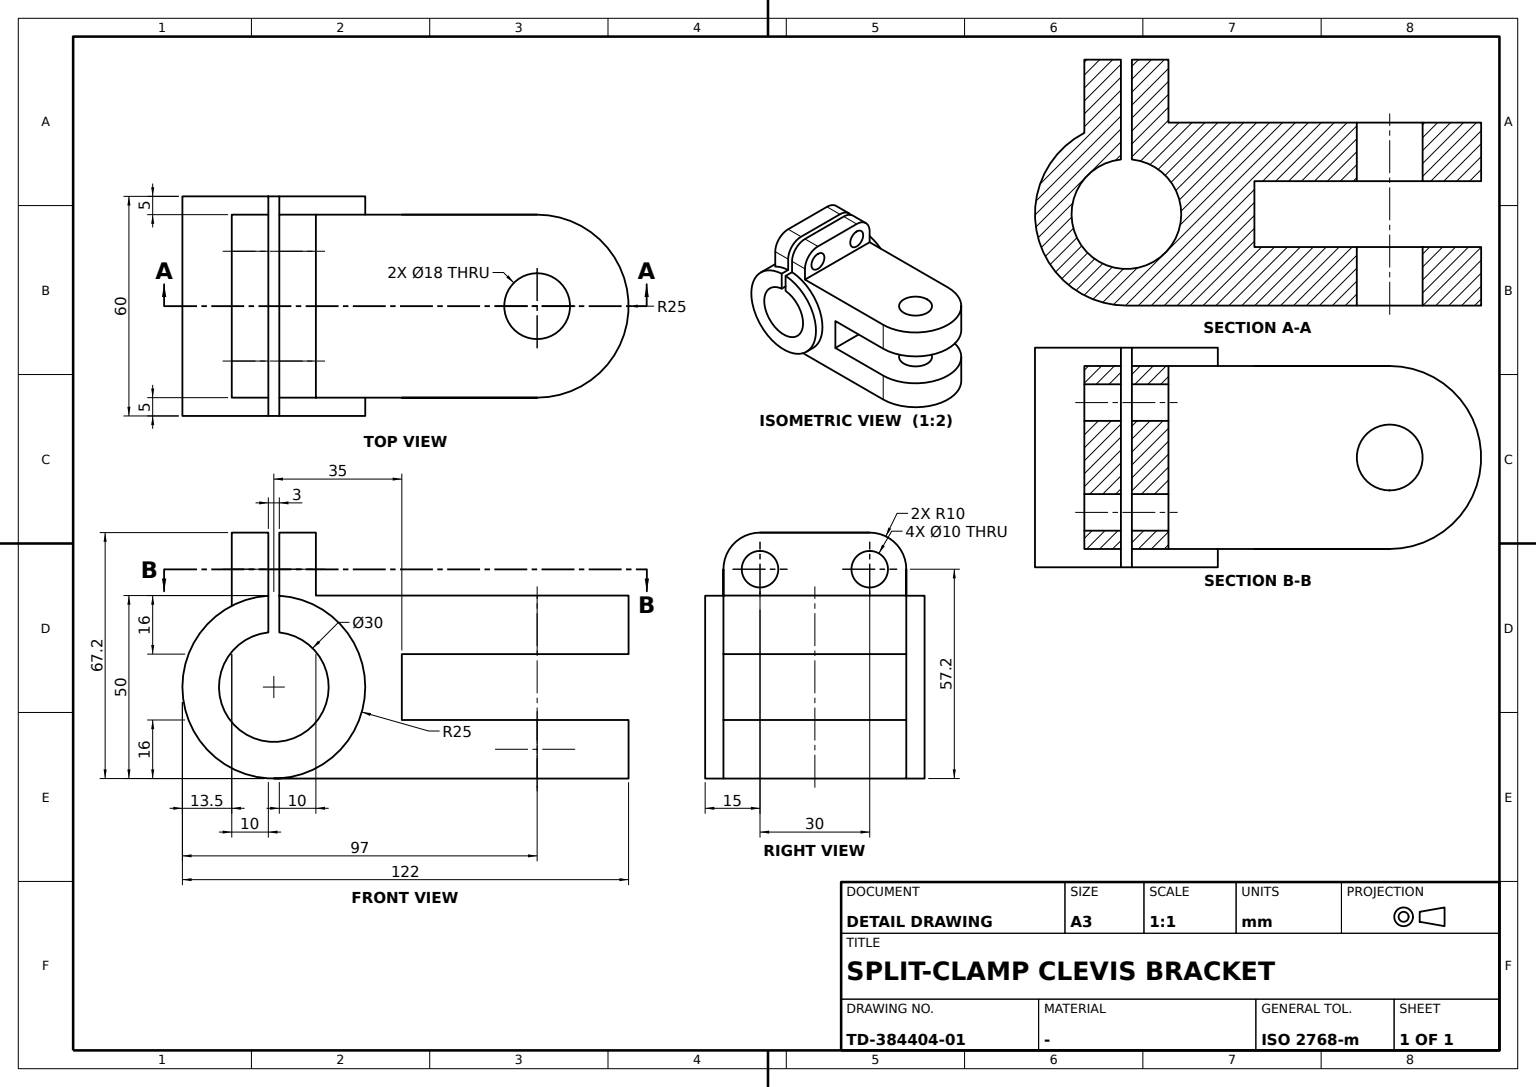
ISO-10303-21;
HEADER;
FILE_DESCRIPTION((''),'2;1');
FILE_NAME('','',(''),(''),'','','');
FILE_SCHEMA(('AUTOMOTIVE_DESIGN'));
ENDSEC;
DATA;
#1=APPLICATION_CONTEXT('');
#2=PRODUCT_CONTEXT('',#1,'mechanical');
#3=PRODUCT('','','',(#2));
#4=PRODUCT_DEFINITION_FORMATION('','',#3);
#5=PRODUCT_DEFINITION_CONTEXT('',#1,'design');
#6=PRODUCT_DEFINITION('','',#4,#5);
#7=PRODUCT_DEFINITION_SHAPE('','',#6);
#8=(LENGTH_UNIT()NAMED_UNIT(*)SI_UNIT(.MILLI.,.METRE.));
#9=(NAMED_UNIT(*)PLANE_ANGLE_UNIT()SI_UNIT($,.RADIAN.));
#10=(NAMED_UNIT(*)SI_UNIT($,.STERADIAN.)SOLID_ANGLE_UNIT());
#11=UNCERTAINTY_MEASURE_WITH_UNIT(LENGTH_MEASURE(0.005),#8,'distance_accuracy_value','');
#12=(GEOMETRIC_REPRESENTATION_CONTEXT(3)GLOBAL_UNCERTAINTY_ASSIGNED_CONTEXT((#11))GLOBAL_UNIT_ASSIGNED_CONTEXT((#8,#9,#10))REPRESENTATION_CONTEXT('',''));
#13=CARTESIAN_POINT('',(9.,72.,-25.));
#14=VERTEX_POINT('',#13);
#15=CARTESIAN_POINT('',(0.,72.,-25.));
#16=DIRECTION('',(0.,0.,1.));
#17=DIRECTION('',(1.,0.,0.));
#18=AXIS2_PLACEMENT_3D('',#15,#16,#17);
#19=CIRCLE('',#18,9.);
#20=EDGE_CURVE('',#14,#14,#19,.T.);
#21=ORIENTED_EDGE('',*,*,#20,.T.);
#22=EDGE_LOOP('',(#21));
#23=FACE_BOUND('',#22,.T.);
#24=CARTESIAN_POINT('',(-25.,0.,-25.));
#25=VERTEX_POINT('',#24);
#26=CARTESIAN_POINT('',(25.,0.,-25.));
#27=VERTEX_POINT('',#26);
#28=CARTESIAN_POINT('',(0.,0.,-25.));
#29=VECTOR('',#17,1000.);
#30=LINE('',#28,#29);
#31=EDGE_CURVE('',#25,#27,#30,.T.);
#32=ORIENTED_EDGE('',*,*,#31,.F.);
#33=CARTESIAN_POINT('',(-25.,72.,-25.));
#34=VERTEX_POINT('',#33);
#35=DIRECTION('',(0.,-1.,0.));
#36=VECTOR('',#35,1000.);
#37=LINE('',#24,#36);
#38=EDGE_CURVE('',#34,#25,#37,.T.);
#39=ORIENTED_EDGE('',*,*,#38,.F.);
#40=CARTESIAN_POINT('',(25.,72.,-25.));
#41=VERTEX_POINT('',#40);
#42=CIRCLE('',#18,25.);
#43=EDGE_CURVE('',#41,#34,#42,.T.);
#44=ORIENTED_EDGE('',*,*,#43,.F.);
#45=LINE('',#26,#36);
#46=EDGE_CURVE('',#41,#27,#45,.T.);
#47=ORIENTED_EDGE('',*,*,#46,.T.);
#48=EDGE_LOOP('',(#32,#39,#44,#47));
#49=FACE_BOUND('',#48,.T.);
#50=CARTESIAN_POINT('',(0.,97.,-25.));
#51=AXIS2_PLACEMENT_3D('',#50,#16,#35);
#52=PLANE('',#51);
#53=ADVANCED_FACE('',(#23,#49),#52,.F.);
#54=CARTESIAN_POINT('',(25.,-1.5,24.954959));
#55=VERTEX_POINT('',#54);
#56=CARTESIAN_POINT('',(25.,-11.5,22.197973));
#57=VERTEX_POINT('',#56);
#58=CARTESIAN_POINT('',(25.,0.,0.));
#59=DIRECTION('',(0.,0.,-1.));
#60=AXIS2_PLACEMENT_3D('',#58,#17,#59);
#61=CIRCLE('',#60,25.);
#62=EDGE_CURVE('',#55,#57,#61,.T.);
#63=ORIENTED_EDGE('',*,*,#62,.F.);
#64=CARTESIAN_POINT('',(25.,-1.5,32.197973));
#65=VERTEX_POINT('',#64);
#66=CARTESIAN_POINT('',(25.,-1.5,0.));
#67=VECTOR('',#16,1000.);
#68=LINE('',#66,#67);
#69=EDGE_CURVE('',#55,#65,#68,.T.);
#70=ORIENTED_EDGE('',*,*,#69,.T.);
#71=CARTESIAN_POINT('',(25.,-11.5,32.197973));
#72=VERTEX_POINT('',#71);
#73=CARTESIAN_POINT('',(25.,-6.5,32.197973));
#74=DIRECTION('',(0.,1.,0.));
#75=VECTOR('',#74,1000.);
#76=LINE('',#73,#75);
#77=EDGE_CURVE('',#72,#65,#76,.T.);
#78=ORIENTED_EDGE('',*,*,#77,.F.);
#79=CARTESIAN_POINT('',(25.,-11.5,0.));
#80=VECTOR('',#59,1000.);
#81=LINE('',#79,#80);
#82=EDGE_CURVE('',#72,#57,#81,.T.);
#83=ORIENTED_EDGE('',*,*,#82,.T.);
#84=EDGE_LOOP('',(#63,#70,#78,#83));
#85=FACE_BOUND('',#84,.T.);
#86=AXIS2_PLACEMENT_3D('',#58,#17,#74);
#87=PLANE('',#86);
#88=ADVANCED_FACE('',(#85),#87,.T.);
#89=ORIENTED_EDGE('',*,*,#46,.F.);
#90=CARTESIAN_POINT('',(25.,72.,-9.));
#91=VERTEX_POINT('',#90);
#92=CARTESIAN_POINT('',(25.,72.,8.598986));
#93=LINE('',#92,#80);
#94=EDGE_CURVE('',#91,#41,#93,.T.);
#95=ORIENTED_EDGE('',*,*,#94,.F.);
#96=CARTESIAN_POINT('',(25.,35.,-9.));
#97=VERTEX_POINT('',#96);
#98=CARTESIAN_POINT('',(25.,0.,-9.));
#99=LINE('',#98,#75);
#100=EDGE_CURVE('',#97,#91,#99,.T.);
#101=ORIENTED_EDGE('',*,*,#100,.F.);
#102=CARTESIAN_POINT('',(25.,35.,9.));
#103=VERTEX_POINT('',#102);
#104=CARTESIAN_POINT('',(25.,35.,0.));
#105=LINE('',#104,#80);
#106=EDGE_CURVE('',#103,#97,#105,.T.);
#107=ORIENTED_EDGE('',*,*,#106,.F.);
#108=CARTESIAN_POINT('',(25.,72.,9.));
#109=VERTEX_POINT('',#108);
#110=CARTESIAN_POINT('',(25.,0.,9.));
#111=LINE('',#110,#36);
#112=EDGE_CURVE('',#109,#103,#111,.T.);
#113=ORIENTED_EDGE('',*,*,#112,.F.);
#114=CARTESIAN_POINT('',(25.,72.,25.));
#115=VERTEX_POINT('',#114);
#116=EDGE_CURVE('',#115,#109,#93,.T.);
#117=ORIENTED_EDGE('',*,*,#116,.F.);
#118=CARTESIAN_POINT('',(25.,11.5,25.));
#119=VERTEX_POINT('',#118);
#120=CARTESIAN_POINT('',(25.,0.,25.));
#121=LINE('',#120,#75);
#122=EDGE_CURVE('',#119,#115,#121,.T.);
#123=ORIENTED_EDGE('',*,*,#122,.F.);
#124=CARTESIAN_POINT('',(25.,11.5,32.197973));
#125=VERTEX_POINT('',#124);
#126=CARTESIAN_POINT('',(25.,11.5,0.));
#127=LINE('',#126,#80);
#128=EDGE_CURVE('',#125,#119,#127,.T.);
#129=ORIENTED_EDGE('',*,*,#128,.F.);
#130=CARTESIAN_POINT('',(25.,1.5,32.197969));
#131=VERTEX_POINT('',#130);
#132=EDGE_CURVE('',#125,#131,#76,.F.);
#133=ORIENTED_EDGE('',*,*,#132,.T.);
#134=CARTESIAN_POINT('',(25.,1.5,24.954959));
#135=VERTEX_POINT('',#134);
#136=CARTESIAN_POINT('',(25.,1.5,0.));
#137=LINE('',#136,#67);
#138=EDGE_CURVE('',#135,#131,#137,.T.);
#139=ORIENTED_EDGE('',*,*,#138,.F.);
#140=EDGE_CURVE('',#27,#135,#61,.T.);
#141=ORIENTED_EDGE('',*,*,#140,.F.);
#142=EDGE_LOOP('',(#89,#95,#101,#107,#113,#117,#123,#129,#133,#139,#141));
#143=FACE_BOUND('',#142,.T.);
#144=ADVANCED_FACE('',(#143),#87,.T.);
#145=ORIENTED_EDGE('',*,*,#94,.T.);
#146=ORIENTED_EDGE('',*,*,#43,.T.);
#147=CARTESIAN_POINT('',(-25.,72.,-9.));
#148=VERTEX_POINT('',#147);
#149=CARTESIAN_POINT('',(-25.,72.,8.598986));
#150=LINE('',#149,#80);
#151=EDGE_CURVE('',#148,#34,#150,.T.);
#152=ORIENTED_EDGE('',*,*,#151,.F.);
#153=CARTESIAN_POINT('',(0.,72.,-9.));
#154=DIRECTION('',(-1.,0.,0.));
#155=AXIS2_PLACEMENT_3D('',#153,#59,#154);
#156=CIRCLE('',#155,25.);
#157=EDGE_CURVE('',#148,#91,#156,.T.);
#158=ORIENTED_EDGE('',*,*,#157,.T.);
#159=EDGE_LOOP('',(#145,#146,#152,#158));
#160=FACE_BOUND('',#159,.T.);
#161=CARTESIAN_POINT('',(0.,72.,8.598986));
#162=AXIS2_PLACEMENT_3D('',#161,#59,#74);
#163=CYLINDRICAL_SURFACE('',#162,25.);
#164=ADVANCED_FACE('',(#160),#163,.T.);
#165=CARTESIAN_POINT('',(-25.,35.,9.));
#166=VERTEX_POINT('',#165);
#167=CARTESIAN_POINT('',(-25.,35.,-9.));
#168=VERTEX_POINT('',#167);
#169=CARTESIAN_POINT('',(-25.,35.,0.));
#170=LINE('',#169,#80);
#171=EDGE_CURVE('',#166,#168,#170,.T.);
#172=ORIENTED_EDGE('',*,*,#171,.F.);
#173=CARTESIAN_POINT('',(0.,35.,9.));
#174=LINE('',#173,#29);
#175=EDGE_CURVE('',#166,#103,#174,.T.);
#176=ORIENTED_EDGE('',*,*,#175,.T.);
#177=ORIENTED_EDGE('',*,*,#106,.T.);
#178=CARTESIAN_POINT('',(0.,35.,-9.));
#179=LINE('',#178,#29);
#180=EDGE_CURVE('',#168,#97,#179,.T.);
#181=ORIENTED_EDGE('',*,*,#180,.F.);
#182=EDGE_LOOP('',(#172,#176,#177,#181));
#183=FACE_BOUND('',#182,.T.);
#184=AXIS2_PLACEMENT_3D('',#173,#35,#59);
#185=PLANE('',#184);
#186=ADVANCED_FACE('',(#183),#185,.F.);
#187=CARTESIAN_POINT('',(-15.,-11.5,42.197973));
#188=VERTEX_POINT('',#187);
#189=CARTESIAN_POINT('',(15.,-11.5,42.197973));
#190=VERTEX_POINT('',#189);
#191=CARTESIAN_POINT('',(0.,-11.5,42.197973));
#192=LINE('',#191,#29);
#193=EDGE_CURVE('',#188,#190,#192,.T.);
#194=ORIENTED_EDGE('',*,*,#193,.T.);
#195=CARTESIAN_POINT('',(15.,-1.5,42.197973));
#196=VERTEX_POINT('',#195);
#197=CARTESIAN_POINT('',(15.,-6.5,42.197973));
#198=LINE('',#197,#75);
#199=EDGE_CURVE('',#190,#196,#198,.T.);
#200=ORIENTED_EDGE('',*,*,#199,.T.);
#201=CARTESIAN_POINT('',(-15.,-1.5,42.197973));
#202=VERTEX_POINT('',#201);
#203=CARTESIAN_POINT('',(0.,-1.5,42.197973));
#204=LINE('',#203,#29);
#205=EDGE_CURVE('',#202,#196,#204,.T.);
#206=ORIENTED_EDGE('',*,*,#205,.F.);
#207=CARTESIAN_POINT('',(-15.,-6.5,42.197973));
#208=LINE('',#207,#36);
#209=EDGE_CURVE('',#202,#188,#208,.T.);
#210=ORIENTED_EDGE('',*,*,#209,.T.);
#211=EDGE_LOOP('',(#194,#200,#206,#210));
#212=FACE_BOUND('',#211,.T.);
#213=AXIS2_PLACEMENT_3D('',#203,#16,#35);
#214=PLANE('',#213);
#215=ADVANCED_FACE('',(#212),#214,.T.);
#216=CARTESIAN_POINT('',(-15.,11.5,27.197973));
#217=VERTEX_POINT('',#216);
#218=CARTESIAN_POINT('',(-15.,11.5,32.197973));
#219=AXIS2_PLACEMENT_3D('',#218,#35,#59);
#220=CIRCLE('',#219,5.);
#221=EDGE_CURVE('',#217,#217,#220,.F.);
#222=ORIENTED_EDGE('',*,*,#221,.F.);
#223=EDGE_LOOP('',(#222));
#224=FACE_BOUND('',#223,.T.);
#225=CARTESIAN_POINT('',(-25.,11.5,32.197969));
#226=VERTEX_POINT('',#225);
#227=CARTESIAN_POINT('',(-25.,11.5,25.));
#228=VERTEX_POINT('',#227);
#229=CARTESIAN_POINT('',(-25.,11.5,0.));
#230=LINE('',#229,#80);
#231=EDGE_CURVE('',#226,#228,#230,.T.);
#232=ORIENTED_EDGE('',*,*,#231,.F.);
#233=CARTESIAN_POINT('',(-15.,11.5,42.197973));
#234=VERTEX_POINT('',#233);
#235=CIRCLE('',#219,10.);
#236=EDGE_CURVE('',#234,#226,#235,.T.);
#237=ORIENTED_EDGE('',*,*,#236,.F.);
#238=CARTESIAN_POINT('',(14.999996,11.5,42.197973));
#239=VERTEX_POINT('',#238);
#240=CARTESIAN_POINT('',(0.,11.5,42.197973));
#241=LINE('',#240,#29);
#242=EDGE_CURVE('',#234,#239,#241,.T.);
#243=ORIENTED_EDGE('',*,*,#242,.T.);
#244=CARTESIAN_POINT('',(15.,11.5,32.197973));
#245=AXIS2_PLACEMENT_3D('',#244,#35,#59);
#246=CIRCLE('',#245,10.);
#247=EDGE_CURVE('',#125,#239,#246,.T.);
#248=ORIENTED_EDGE('',*,*,#247,.F.);
#249=ORIENTED_EDGE('',*,*,#128,.T.);
#250=CARTESIAN_POINT('',(0.,11.5,25.));
#251=LINE('',#250,#29);
#252=EDGE_CURVE('',#228,#119,#251,.T.);
#253=ORIENTED_EDGE('',*,*,#252,.F.);
#254=EDGE_LOOP('',(#232,#237,#243,#248,#249,#253));
#255=FACE_BOUND('',#254,.T.);
#256=CARTESIAN_POINT('',(15.,11.5,27.197973));
#257=VERTEX_POINT('',#256);
#258=CIRCLE('',#245,5.);
#259=EDGE_CURVE('',#257,#257,#258,.F.);
#260=ORIENTED_EDGE('',*,*,#259,.F.);
#261=EDGE_LOOP('',(#260));
#262=FACE_BOUND('',#261,.T.);
#263=AXIS2_PLACEMENT_3D('',#240,#35,#59);
#264=PLANE('',#263);
#265=ADVANCED_FACE('',(#224,#255,#262),#264,.F.);
#266=CARTESIAN_POINT('',(-30.,1.5,14.924812));
#267=VERTEX_POINT('',#266);
#268=CARTESIAN_POINT('',(-30.,1.5,24.954959));
#269=VERTEX_POINT('',#268);
#270=CARTESIAN_POINT('',(-30.,1.5,0.));
#271=LINE('',#270,#67);
#272=EDGE_CURVE('',#267,#269,#271,.T.);
#273=ORIENTED_EDGE('',*,*,#272,.T.);
#274=CARTESIAN_POINT('',(-30.,-1.5,24.954959));
#275=VERTEX_POINT('',#274);
#276=CARTESIAN_POINT('',(-30.,0.,0.));
#277=AXIS2_PLACEMENT_3D('',#276,#17,#59);
#278=CIRCLE('',#277,25.);
#279=EDGE_CURVE('',#275,#269,#278,.T.);
#280=ORIENTED_EDGE('',*,*,#279,.F.);
#281=CARTESIAN_POINT('',(-30.,-1.5,14.924812));
#282=VERTEX_POINT('',#281);
#283=CARTESIAN_POINT('',(-30.,-1.5,0.));
#284=LINE('',#283,#67);
#285=EDGE_CURVE('',#282,#275,#284,.T.);
#286=ORIENTED_EDGE('',*,*,#285,.F.);
#287=CIRCLE('',#277,15.);
#288=EDGE_CURVE('',#282,#267,#287,.T.);
#289=ORIENTED_EDGE('',*,*,#288,.T.);
#290=EDGE_LOOP('',(#273,#280,#286,#289));
#291=FACE_BOUND('',#290,.T.);
#292=AXIS2_PLACEMENT_3D('',#276,#17,#74);
#293=PLANE('',#292);
#294=ADVANCED_FACE('',(#291),#293,.F.);
#295=CARTESIAN_POINT('',(-9.,72.,25.));
#296=VERTEX_POINT('',#295);
#297=CARTESIAN_POINT('',(0.,72.,25.));
#298=AXIS2_PLACEMENT_3D('',#297,#59,#154);
#299=CIRCLE('',#298,9.);
#300=EDGE_CURVE('',#296,#296,#299,.F.);
#301=ORIENTED_EDGE('',*,*,#300,.F.);
#302=EDGE_LOOP('',(#301));
#303=FACE_BOUND('',#302,.T.);
#304=ORIENTED_EDGE('',*,*,#252,.T.);
#305=ORIENTED_EDGE('',*,*,#122,.T.);
#306=CARTESIAN_POINT('',(-25.,72.,25.));
#307=VERTEX_POINT('',#306);
#308=CIRCLE('',#298,25.);
#309=EDGE_CURVE('',#307,#115,#308,.T.);
#310=ORIENTED_EDGE('',*,*,#309,.F.);
#311=CARTESIAN_POINT('',(-25.,0.,25.));
#312=LINE('',#311,#75);
#313=EDGE_CURVE('',#228,#307,#312,.T.);
#314=ORIENTED_EDGE('',*,*,#313,.F.);
#315=EDGE_LOOP('',(#304,#305,#310,#314));
#316=FACE_BOUND('',#315,.T.);
#317=AXIS2_PLACEMENT_3D('',#250,#59,#74);
#318=PLANE('',#317);
#319=ADVANCED_FACE('',(#303,#316),#318,.F.);
#320=CARTESIAN_POINT('',(15.,-1.5,32.197973));
#321=AXIS2_PLACEMENT_3D('',#320,#74,#16);
#322=CIRCLE('',#321,10.);
#323=EDGE_CURVE('',#196,#65,#322,.T.);
#324=ORIENTED_EDGE('',*,*,#323,.T.);
#325=ORIENTED_EDGE('',*,*,#69,.F.);
#326=CARTESIAN_POINT('',(30.,-1.5,24.954959));
#327=VERTEX_POINT('',#326);
#328=LINE('',#54,#29);
#329=EDGE_CURVE('',#55,#327,#328,.T.);
#330=ORIENTED_EDGE('',*,*,#329,.T.);
#331=CARTESIAN_POINT('',(30.,-1.5,14.924812));
#332=VERTEX_POINT('',#331);
#333=CARTESIAN_POINT('',(30.,-1.5,0.));
#334=LINE('',#333,#67);
#335=EDGE_CURVE('',#332,#327,#334,.T.);
#336=ORIENTED_EDGE('',*,*,#335,.F.);
#337=LINE('',#281,#29);
#338=EDGE_CURVE('',#282,#332,#337,.T.);
#339=ORIENTED_EDGE('',*,*,#338,.F.);
#340=ORIENTED_EDGE('',*,*,#285,.T.);
#341=CARTESIAN_POINT('',(-25.,-1.5,24.954959));
#342=VERTEX_POINT('',#341);
#343=LINE('',#274,#29);
#344=EDGE_CURVE('',#275,#342,#343,.T.);
#345=ORIENTED_EDGE('',*,*,#344,.T.);
#346=CARTESIAN_POINT('',(-25.,-1.5,32.197973));
#347=VERTEX_POINT('',#346);
#348=CARTESIAN_POINT('',(-25.,-1.5,0.));
#349=LINE('',#348,#67);
#350=EDGE_CURVE('',#342,#347,#349,.T.);
#351=ORIENTED_EDGE('',*,*,#350,.T.);
#352=CARTESIAN_POINT('',(-15.,-1.5,32.197973));
#353=AXIS2_PLACEMENT_3D('',#352,#74,#16);
#354=CIRCLE('',#353,10.);
#355=EDGE_CURVE('',#347,#202,#354,.T.);
#356=ORIENTED_EDGE('',*,*,#355,.T.);
#357=ORIENTED_EDGE('',*,*,#205,.T.);
#358=EDGE_LOOP('',(#324,#325,#330,#336,#339,#340,#345,#351,#356,#357));
#359=FACE_BOUND('',#358,.T.);
#360=CARTESIAN_POINT('',(15.,-1.5,37.197973));
#361=VERTEX_POINT('',#360);
#362=CIRCLE('',#321,5.);
#363=EDGE_CURVE('',#361,#361,#362,.T.);
#364=ORIENTED_EDGE('',*,*,#363,.F.);
#365=EDGE_LOOP('',(#364));
#366=FACE_BOUND('',#365,.T.);
#367=CARTESIAN_POINT('',(-15.,-1.5,37.197973));
#368=VERTEX_POINT('',#367);
#369=CIRCLE('',#353,5.);
#370=EDGE_CURVE('',#368,#368,#369,.T.);
#371=ORIENTED_EDGE('',*,*,#370,.F.);
#372=EDGE_LOOP('',(#371));
#373=FACE_BOUND('',#372,.T.);
#374=CARTESIAN_POINT('',(0.,-1.5,14.924812));
#375=AXIS2_PLACEMENT_3D('',#374,#74,#16);
#376=PLANE('',#375);
#377=ADVANCED_FACE('',(#359,#366,#373),#376,.T.);
#378=ORIENTED_EDGE('',*,*,#20,.F.);
#379=EDGE_LOOP('',(#378));
#380=FACE_BOUND('',#379,.T.);
#381=CARTESIAN_POINT('',(-9.,72.,-9.));
#382=VERTEX_POINT('',#381);
#383=CIRCLE('',#155,9.);
#384=EDGE_CURVE('',#382,#382,#383,.T.);
#385=ORIENTED_EDGE('',*,*,#384,.F.);
#386=EDGE_LOOP('',(#385));
#387=FACE_BOUND('',#386,.T.);
#388=CARTESIAN_POINT('',(0.,72.,-0.66));
#389=AXIS2_PLACEMENT_3D('',#388,#16,#17);
#390=CYLINDRICAL_SURFACE('',#389,9.);
#391=ADVANCED_FACE('',(#380,#387),#390,.F.);
#392=ORIENTED_EDGE('',*,*,#309,.T.);
#393=ORIENTED_EDGE('',*,*,#116,.T.);
#394=CARTESIAN_POINT('',(-25.,72.,9.));
#395=VERTEX_POINT('',#394);
#396=CARTESIAN_POINT('',(0.,72.,9.));
#397=AXIS2_PLACEMENT_3D('',#396,#16,#17);
#398=CIRCLE('',#397,25.);
#399=EDGE_CURVE('',#109,#395,#398,.T.);
#400=ORIENTED_EDGE('',*,*,#399,.T.);
#401=EDGE_CURVE('',#307,#395,#150,.T.);
#402=ORIENTED_EDGE('',*,*,#401,.F.);
#403=EDGE_LOOP('',(#392,#393,#400,#402));
#404=FACE_BOUND('',#403,.T.);
#405=ADVANCED_FACE('',(#404),#163,.T.);
#406=CARTESIAN_POINT('',(30.,1.5,14.924812));
#407=VERTEX_POINT('',#406);
#408=CARTESIAN_POINT('',(30.,0.,0.));
#409=AXIS2_PLACEMENT_3D('',#408,#17,#59);
#410=CIRCLE('',#409,15.);
#411=EDGE_CURVE('',#332,#407,#410,.T.);
#412=ORIENTED_EDGE('',*,*,#411,.T.);
#413=LINE('',#266,#29);
#414=EDGE_CURVE('',#267,#407,#413,.T.);
#415=ORIENTED_EDGE('',*,*,#414,.F.);
#416=ORIENTED_EDGE('',*,*,#288,.F.);
#417=ORIENTED_EDGE('',*,*,#338,.T.);
#418=EDGE_LOOP('',(#412,#415,#416,#417));
#419=FACE_BOUND('',#418,.T.);
#420=CARTESIAN_POINT('',(0.,0.,0.));
#421=AXIS2_PLACEMENT_3D('',#420,#17,#74);
#422=CYLINDRICAL_SURFACE('',#421,15.);
#423=ADVANCED_FACE('',(#419),#422,.F.);
#424=CARTESIAN_POINT('',(-25.,-11.5,22.197973));
#425=VERTEX_POINT('',#424);
#426=CARTESIAN_POINT('',(-25.,0.,0.));
#427=AXIS2_PLACEMENT_3D('',#426,#17,#59);
#428=CIRCLE('',#427,25.);
#429=EDGE_CURVE('',#342,#425,#428,.T.);
#430=ORIENTED_EDGE('',*,*,#429,.F.);
#431=ORIENTED_EDGE('',*,*,#344,.F.);
#432=ORIENTED_EDGE('',*,*,#279,.T.);
#433=CARTESIAN_POINT('',(-25.,1.5,24.954959));
#434=VERTEX_POINT('',#433);
#435=LINE('',#268,#29);
#436=EDGE_CURVE('',#269,#434,#435,.T.);
#437=ORIENTED_EDGE('',*,*,#436,.T.);
#438=EDGE_CURVE('',#25,#434,#428,.T.);
#439=ORIENTED_EDGE('',*,*,#438,.F.);
#440=ORIENTED_EDGE('',*,*,#31,.T.);
#441=ORIENTED_EDGE('',*,*,#140,.T.);
#442=CARTESIAN_POINT('',(30.,1.5,24.954959));
#443=VERTEX_POINT('',#442);
#444=LINE('',#134,#29);
#445=EDGE_CURVE('',#135,#443,#444,.T.);
#446=ORIENTED_EDGE('',*,*,#445,.T.);
#447=CIRCLE('',#409,25.);
#448=EDGE_CURVE('',#327,#443,#447,.T.);
#449=ORIENTED_EDGE('',*,*,#448,.F.);
#450=ORIENTED_EDGE('',*,*,#329,.F.);
#451=ORIENTED_EDGE('',*,*,#62,.T.);
#452=LINE('',#424,#29);
#453=EDGE_CURVE('',#425,#57,#452,.T.);
#454=ORIENTED_EDGE('',*,*,#453,.F.);
#455=EDGE_LOOP('',(#430,#431,#432,#437,#439,#440,#441,#446,#449,#450,#451,#454));
#456=FACE_BOUND('',#455,.T.);
#457=CYLINDRICAL_SURFACE('',#421,25.);
#458=ADVANCED_FACE('',(#456),#457,.T.);
#459=CARTESIAN_POINT('',(-14.999996,1.5,42.197973));
#460=VERTEX_POINT('',#459);
#461=CARTESIAN_POINT('',(15.,1.5,42.197973));
#462=VERTEX_POINT('',#461);
#463=CARTESIAN_POINT('',(0.,1.5,42.197973));
#464=LINE('',#463,#29);
#465=EDGE_CURVE('',#460,#462,#464,.T.);
#466=ORIENTED_EDGE('',*,*,#465,.T.);
#467=EDGE_CURVE('',#239,#462,#198,.F.);
#468=ORIENTED_EDGE('',*,*,#467,.F.);
#469=ORIENTED_EDGE('',*,*,#242,.F.);
#470=EDGE_CURVE('',#234,#460,#208,.T.);
#471=ORIENTED_EDGE('',*,*,#470,.T.);
#472=EDGE_LOOP('',(#466,#468,#469,#471));
#473=FACE_BOUND('',#472,.T.);
#474=ADVANCED_FACE('',(#473),#214,.T.);
#475=ORIENTED_EDGE('',*,*,#175,.F.);
#476=CARTESIAN_POINT('',(-25.,0.,9.));
#477=LINE('',#476,#36);
#478=EDGE_CURVE('',#395,#166,#477,.T.);
#479=ORIENTED_EDGE('',*,*,#478,.F.);
#480=ORIENTED_EDGE('',*,*,#399,.F.);
#481=ORIENTED_EDGE('',*,*,#112,.T.);
#482=EDGE_LOOP('',(#475,#479,#480,#481));
#483=FACE_BOUND('',#482,.T.);
#484=CARTESIAN_POINT('',(9.,72.,9.));
#485=VERTEX_POINT('',#484);
#486=CIRCLE('',#397,9.);
#487=EDGE_CURVE('',#485,#485,#486,.T.);
#488=ORIENTED_EDGE('',*,*,#487,.T.);
#489=EDGE_LOOP('',(#488));
#490=FACE_BOUND('',#489,.T.);
#491=CARTESIAN_POINT('',(0.,97.,9.));
#492=AXIS2_PLACEMENT_3D('',#491,#16,#35);
#493=PLANE('',#492);
#494=ADVANCED_FACE('',(#483,#490),#493,.F.);
#495=CARTESIAN_POINT('',(-15.,-11.5,27.197973));
#496=VERTEX_POINT('',#495);
#497=CARTESIAN_POINT('',(-15.,-11.5,32.197973));
#498=AXIS2_PLACEMENT_3D('',#497,#35,#59);
#499=CIRCLE('',#498,5.);
#500=EDGE_CURVE('',#496,#496,#499,.T.);
#501=ORIENTED_EDGE('',*,*,#500,.T.);
#502=EDGE_LOOP('',(#501));
#503=FACE_BOUND('',#502,.T.);
#504=ORIENTED_EDGE('',*,*,#370,.T.);
#505=EDGE_LOOP('',(#504));
#506=FACE_BOUND('',#505,.T.);
#507=CARTESIAN_POINT('',(-15.,-7.41,32.197973));
#508=AXIS2_PLACEMENT_3D('',#507,#74,#154);
#509=CYLINDRICAL_SURFACE('',#508,5.);
#510=ADVANCED_FACE('',(#503,#506),#509,.F.);
#511=CARTESIAN_POINT('',(-25.,1.5,32.197973));
#512=VERTEX_POINT('',#511);
#513=CARTESIAN_POINT('',(-15.,1.5,32.197973));
#514=AXIS2_PLACEMENT_3D('',#513,#74,#16);
#515=CIRCLE('',#514,10.);
#516=EDGE_CURVE('',#512,#460,#515,.T.);
#517=ORIENTED_EDGE('',*,*,#516,.T.);
#518=ORIENTED_EDGE('',*,*,#470,.F.);
#519=ORIENTED_EDGE('',*,*,#236,.T.);
#520=CARTESIAN_POINT('',(-25.,-6.5,32.197973));
#521=LINE('',#520,#36);
#522=EDGE_CURVE('',#226,#512,#521,.T.);
#523=ORIENTED_EDGE('',*,*,#522,.T.);
#524=EDGE_LOOP('',(#517,#518,#519,#523));
#525=FACE_BOUND('',#524,.T.);
#526=CARTESIAN_POINT('',(-15.,-6.5,32.197973));
#527=AXIS2_PLACEMENT_3D('',#526,#35,#154);
#528=CYLINDRICAL_SURFACE('',#527,10.);
#529=ADVANCED_FACE('',(#525),#528,.T.);
#530=ORIENTED_EDGE('',*,*,#355,.F.);
#531=CARTESIAN_POINT('',(-25.,-11.5,32.197973));
#532=VERTEX_POINT('',#531);
#533=EDGE_CURVE('',#347,#532,#521,.T.);
#534=ORIENTED_EDGE('',*,*,#533,.T.);
#535=CIRCLE('',#498,10.);
#536=EDGE_CURVE('',#188,#532,#535,.T.);
#537=ORIENTED_EDGE('',*,*,#536,.F.);
#538=ORIENTED_EDGE('',*,*,#209,.F.);
#539=EDGE_LOOP('',(#530,#534,#537,#538));
#540=FACE_BOUND('',#539,.T.);
#541=ADVANCED_FACE('',(#540),#528,.T.);
#542=CARTESIAN_POINT('',(-15.,1.5,37.197973));
#543=VERTEX_POINT('',#542);
#544=CIRCLE('',#514,5.);
#545=EDGE_CURVE('',#543,#543,#544,.T.);
#546=ORIENTED_EDGE('',*,*,#545,.T.);
#547=EDGE_LOOP('',(#546));
#548=FACE_BOUND('',#547,.T.);
#549=CARTESIAN_POINT('',(15.,1.5,37.197973));
#550=VERTEX_POINT('',#549);
#551=CARTESIAN_POINT('',(15.,1.5,32.197973));
#552=AXIS2_PLACEMENT_3D('',#551,#74,#16);
#553=CIRCLE('',#552,5.);
#554=EDGE_CURVE('',#550,#550,#553,.T.);
#555=ORIENTED_EDGE('',*,*,#554,.T.);
#556=EDGE_LOOP('',(#555));
#557=FACE_BOUND('',#556,.T.);
#558=CARTESIAN_POINT('',(-25.,1.5,0.));
#559=LINE('',#558,#67);
#560=EDGE_CURVE('',#434,#512,#559,.T.);
#561=ORIENTED_EDGE('',*,*,#560,.F.);
#562=ORIENTED_EDGE('',*,*,#436,.F.);
#563=ORIENTED_EDGE('',*,*,#272,.F.);
#564=ORIENTED_EDGE('',*,*,#414,.T.);
#565=CARTESIAN_POINT('',(30.,1.5,0.));
#566=LINE('',#565,#67);
#567=EDGE_CURVE('',#407,#443,#566,.T.);
#568=ORIENTED_EDGE('',*,*,#567,.T.);
#569=ORIENTED_EDGE('',*,*,#445,.F.);
#570=ORIENTED_EDGE('',*,*,#138,.T.);
#571=CIRCLE('',#552,10.);
#572=EDGE_CURVE('',#462,#131,#571,.T.);
#573=ORIENTED_EDGE('',*,*,#572,.F.);
#574=ORIENTED_EDGE('',*,*,#465,.F.);
#575=ORIENTED_EDGE('',*,*,#516,.F.);
#576=EDGE_LOOP('',(#561,#562,#563,#564,#568,#569,#570,#573,#574,#575));
#577=FACE_BOUND('',#576,.T.);
#578=CARTESIAN_POINT('',(0.,1.5,14.924812));
#579=AXIS2_PLACEMENT_3D('',#578,#74,#16);
#580=PLANE('',#579);
#581=ADVANCED_FACE('',(#548,#557,#577),#580,.F.);
#582=ORIENTED_EDGE('',*,*,#77,.T.);
#583=ORIENTED_EDGE('',*,*,#323,.F.);
#584=ORIENTED_EDGE('',*,*,#199,.F.);
#585=CARTESIAN_POINT('',(15.,-11.5,32.197973));
#586=AXIS2_PLACEMENT_3D('',#585,#35,#59);
#587=CIRCLE('',#586,10.);
#588=EDGE_CURVE('',#72,#190,#587,.T.);
#589=ORIENTED_EDGE('',*,*,#588,.F.);
#590=EDGE_LOOP('',(#582,#583,#584,#589));
#591=FACE_BOUND('',#590,.T.);
#592=CARTESIAN_POINT('',(15.,-6.5,32.197973));
#593=AXIS2_PLACEMENT_3D('',#592,#74,#16);
#594=CYLINDRICAL_SURFACE('',#593,10.);
#595=ADVANCED_FACE('',(#591),#594,.T.);
#596=ORIENTED_EDGE('',*,*,#478,.T.);
#597=ORIENTED_EDGE('',*,*,#171,.T.);
#598=CARTESIAN_POINT('',(-25.,0.,-9.));
#599=LINE('',#598,#75);
#600=EDGE_CURVE('',#168,#148,#599,.T.);
#601=ORIENTED_EDGE('',*,*,#600,.T.);
#602=ORIENTED_EDGE('',*,*,#151,.T.);
#603=ORIENTED_EDGE('',*,*,#38,.T.);
#604=ORIENTED_EDGE('',*,*,#438,.T.);
#605=ORIENTED_EDGE('',*,*,#560,.T.);
#606=ORIENTED_EDGE('',*,*,#522,.F.);
#607=ORIENTED_EDGE('',*,*,#231,.T.);
#608=ORIENTED_EDGE('',*,*,#313,.T.);
#609=ORIENTED_EDGE('',*,*,#401,.T.);
#610=EDGE_LOOP('',(#596,#597,#601,#602,#603,#604,#605,#606,#607,#608,#609));
#611=FACE_BOUND('',#610,.T.);
#612=AXIS2_PLACEMENT_3D('',#426,#17,#74);
#613=PLANE('',#612);
#614=ADVANCED_FACE('',(#611),#613,.F.);
#615=CARTESIAN_POINT('',(15.,-11.5,27.197973));
#616=VERTEX_POINT('',#615);
#617=CIRCLE('',#586,5.);
#618=EDGE_CURVE('',#616,#616,#617,.T.);
#619=ORIENTED_EDGE('',*,*,#618,.F.);
#620=EDGE_LOOP('',(#619));
#621=FACE_BOUND('',#620,.T.);
#622=ORIENTED_EDGE('',*,*,#500,.F.);
#623=EDGE_LOOP('',(#622));
#624=FACE_BOUND('',#623,.T.);
#625=ORIENTED_EDGE('',*,*,#82,.F.);
#626=ORIENTED_EDGE('',*,*,#588,.T.);
#627=ORIENTED_EDGE('',*,*,#193,.F.);
#628=ORIENTED_EDGE('',*,*,#536,.T.);
#629=CARTESIAN_POINT('',(-25.,-11.5,0.));
#630=LINE('',#629,#80);
#631=EDGE_CURVE('',#532,#425,#630,.T.);
#632=ORIENTED_EDGE('',*,*,#631,.T.);
#633=ORIENTED_EDGE('',*,*,#453,.T.);
#634=EDGE_LOOP('',(#625,#626,#627,#628,#632,#633));
#635=FACE_BOUND('',#634,.T.);
#636=AXIS2_PLACEMENT_3D('',#191,#35,#59);
#637=PLANE('',#636);
#638=ADVANCED_FACE('',(#621,#624,#635),#637,.T.);
#639=ORIENTED_EDGE('',*,*,#600,.F.);
#640=ORIENTED_EDGE('',*,*,#180,.T.);
#641=ORIENTED_EDGE('',*,*,#100,.T.);
#642=ORIENTED_EDGE('',*,*,#157,.F.);
#643=EDGE_LOOP('',(#639,#640,#641,#642));
#644=FACE_BOUND('',#643,.T.);
#645=ORIENTED_EDGE('',*,*,#384,.T.);
#646=EDGE_LOOP('',(#645));
#647=FACE_BOUND('',#646,.T.);
#648=AXIS2_PLACEMENT_3D('',#178,#59,#74);
#649=PLANE('',#648);
#650=ADVANCED_FACE('',(#644,#647),#649,.F.);
#651=ORIENTED_EDGE('',*,*,#221,.T.);
#652=EDGE_LOOP('',(#651));
#653=FACE_BOUND('',#652,.T.);
#654=ORIENTED_EDGE('',*,*,#545,.F.);
#655=EDGE_LOOP('',(#654));
#656=FACE_BOUND('',#655,.T.);
#657=ADVANCED_FACE('',(#653,#656),#509,.F.);
#658=ORIENTED_EDGE('',*,*,#335,.T.);
#659=ORIENTED_EDGE('',*,*,#448,.T.);
#660=ORIENTED_EDGE('',*,*,#567,.F.);
#661=ORIENTED_EDGE('',*,*,#411,.F.);
#662=EDGE_LOOP('',(#658,#659,#660,#661));
#663=FACE_BOUND('',#662,.T.);
#664=AXIS2_PLACEMENT_3D('',#408,#17,#74);
#665=PLANE('',#664);
#666=ADVANCED_FACE('',(#663),#665,.T.);
#667=ORIENTED_EDGE('',*,*,#554,.F.);
#668=EDGE_LOOP('',(#667));
#669=FACE_BOUND('',#668,.T.);
#670=ORIENTED_EDGE('',*,*,#259,.T.);
#671=EDGE_LOOP('',(#670));
#672=FACE_BOUND('',#671,.T.);
#673=CARTESIAN_POINT('',(15.,-7.41,32.197973));
#674=AXIS2_PLACEMENT_3D('',#673,#74,#154);
#675=CYLINDRICAL_SURFACE('',#674,5.);
#676=ADVANCED_FACE('',(#669,#672),#675,.F.);
#677=ORIENTED_EDGE('',*,*,#300,.T.);
#678=EDGE_LOOP('',(#677));
#679=FACE_BOUND('',#678,.T.);
#680=ORIENTED_EDGE('',*,*,#487,.F.);
#681=EDGE_LOOP('',(#680));
#682=FACE_BOUND('',#681,.T.);
#683=ADVANCED_FACE('',(#679,#682),#390,.F.);
#684=ORIENTED_EDGE('',*,*,#363,.T.);
#685=EDGE_LOOP('',(#684));
#686=FACE_BOUND('',#685,.T.);
#687=ORIENTED_EDGE('',*,*,#618,.T.);
#688=EDGE_LOOP('',(#687));
#689=FACE_BOUND('',#688,.T.);
#690=ADVANCED_FACE('',(#686,#689),#675,.F.);
#691=ORIENTED_EDGE('',*,*,#429,.T.);
#692=ORIENTED_EDGE('',*,*,#631,.F.);
#693=ORIENTED_EDGE('',*,*,#533,.F.);
#694=ORIENTED_EDGE('',*,*,#350,.F.);
#695=EDGE_LOOP('',(#691,#692,#693,#694));
#696=FACE_BOUND('',#695,.T.);
#697=ADVANCED_FACE('',(#696),#613,.F.);
#698=ORIENTED_EDGE('',*,*,#572,.T.);
#699=ORIENTED_EDGE('',*,*,#132,.F.);
#700=ORIENTED_EDGE('',*,*,#247,.T.);
#701=ORIENTED_EDGE('',*,*,#467,.T.);
#702=EDGE_LOOP('',(#698,#699,#700,#701));
#703=FACE_BOUND('',#702,.T.);
#704=ADVANCED_FACE('',(#703),#594,.T.);
#705=CLOSED_SHELL('',(#53,#88,#144,#164,#186,#215,#265,#294,#319,#377,#391,#405,#423,#458,#474,#494,#510,#529,#541,#581,#595,#614,#638,#650,#657,#666,#676,#683,#690,#697,#704));
#706=MANIFOLD_SOLID_BREP('',#705);
#707=ADVANCED_BREP_SHAPE_REPRESENTATION('',(#706),#12);
#708=SHAPE_DEFINITION_REPRESENTATION(#7,#707);
ENDSEC;
END-ISO-10303-21;
